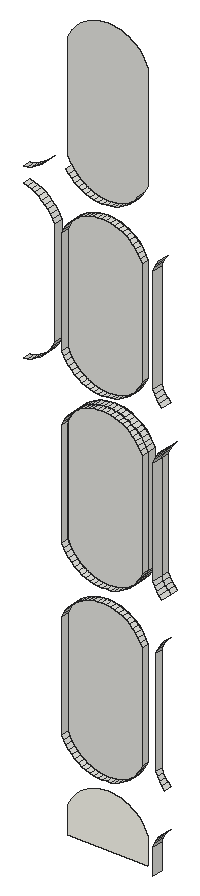
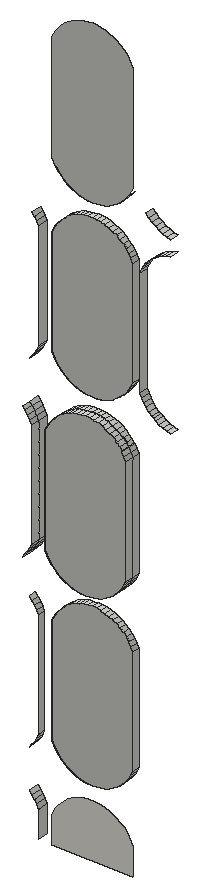
# SketchUp Ruby script. Lengths in inches.
U = 1.inch
M = Sketchup.active_model
def pt(a) = Geom::Point3d.new(a.map { |v| v * U })
def face(e, loops, mat)
  f = e.add_face(loops[0].map { |a| pt(a) })
  loops[1..].each { |l| e.add_face(l.map { |a| pt(a) }).erase! }
  f.material = f.back_material = mat if mat
  f
end
# faces: each face lists its corners as indices into pts; further lists are holes
def faces(e, pts, list, mat = nil) = list.each { |f| face(e, (f[0].is_a?(Array) ? f : [f]).map { |l| l.map { |i| pts[i] } }, mat) }
# xy, xz, yz: faces in a plane at the given z, y or x. An outline is a flat list of corners, or four numbers for a rectangle; further outlines are holes
def ring(l) = l.size == 4 ? [[l[0], l[1]], [l[2], l[1]], [l[2], l[3]], [l[0], l[3]]] : l.each_slice(2).to_a
def flat(e, list, mat, &to3) = list.each { |f| face(e, (f[0].is_a?(Array) ? f : [f]).map { |l| ring(l).map { |u, v| to3.(u, v) } }, mat) }
def xy(e, z, list, mat = nil) = flat(e, list, mat) { |x, y| [x, y, z] }
def xz(e, y, list, mat = nil) = flat(e, list, mat) { |x, z| [x, y, z] }
def yz(e, x, list, mat = nil) = flat(e, list, mat) { |y, z| [x, y, z] }
def lines(e, pts, list) = list.each { |a, b| e.add_line(pt(pts[a]), pt(pts[b])) }
# prism: a flat outline (further loops are holes) pulled along v
def prism(e, loops, v, mat = nil)
  f = face(e, loops, mat); d = Geom::Vector3d.new(v.map { |x| x * U })
  f.pushpull(f.normal.samedirection?(d) ? d.length : -d.length)
end
def box(e, o, s, mat = nil) = prism(e, [[o, [o[0] + s[0], o[1], o[2]], [o[0] + s[0], o[1] + s[1], o[2]], [o[0], o[1] + s[1], o[2]]]], [0, 0, s[2]], mat)
def at(x, y, z, deg = 0) = Geom::Transformation.translation(pt([x, y, z])) * Geom::Transformation.rotation(ORIGIN, Z_AXIS, deg.degrees)
def axes(o, x, y, z) = Geom::Transformation.new([*x, 0, *y, 0, *z, 0, *pt(o).to_a, 1])
def part(name) = M.definitions.add(name)
# library, detail: a bought-in or finely detailed component or shape, given as its bounding box
def library(name, o, s) = part(name).tap { |d| box(d.entities, o, s) }
def detail(e, o, s) = box(e.add_group.entities, o, s)
def put(e, d, t, mat = nil) = e.add_instance(d, t).tap { |i| i.material = mat if mat }
def group(e, t, mat = nil) = e.add_group.tap { |g| g.transformation = t; g.material = mat if mat }.entities
root = M.entities
M.materials.add("Tafisa-Gardenia-or-Gardenia-PM775-4K").color = [246, 245, 235]
xz(root,138.79,[[89.53,11,89.85,11.02,90.17,11.0625,90.48,11.14,90.78,11.25,91.07,11.38,91.35,11.55,91.61,11.73,91.84,11.95,92.0625,12.18,92.25,12.4375,92.42,12.71,92.5625,13,92.5625,21,92.42,21.29,92.25,21.5625,92.0625,21.82,91.84,22.05,91.61,22.27,91.35,22.45,91.07,22.62,90.78,22.75,90.48,22.86,90.17,22.9375,89.85,22.98,89.53,23,89.21,22.98,88.89,22.9375,88.58,22.86,88.28,22.75,87.99,22.62,87.72,22.45,87.46,22.27,87.22,22.05,87,21.82,86.81,21.5625,86.64,21.29,86.5,21,86.5,13,86.64,12.71,86.81,12.4375,87,12.18,87.22,11.95,87.46,11.73,87.72,11.55,87.99,11.38,88.28,11.25,88.58,11.14,88.89,11.0625,89.21,11.02],[89.53,24,89.85,24.02,90.17,24.0625,90.48,24.14,90.78,24.25,91.07,24.38,91.35,24.55,91.61,24.73,91.84,24.95,92.0625,25.18,92.25,25.4375,92.42,25.71,92.5625,26,92.5625,34,92.42,34.29,92.25,34.5625,92.0625,34.82,91.84,35.05,91.61,35.27,91.35,35.45,91.07,35.62,90.78,35.75,90.48,35.86,90.17,35.9375,89.85,35.98,89.53,36,89.21,35.98,88.89,35.9375,88.58,35.86,88.28,35.75,87.99,35.62,87.72,35.45,87.46,35.27,87.22,35.05,87,34.82,86.86,34.63,86.81,34.5625,86.64,34.29,86.5,34,86.5,26,86.64,25.71,86.81,25.4375,87,25.18,87.22,24.95,87.46,24.73,87.72,24.55,87.99,24.38,88.28,24.25,88.58,24.14,88.89,24.0625,89.21,24.02],[89.53,37,89.85,37.02,90.17,37.0625,90.48,37.14,90.78,37.25,91.07,37.38,91.35,37.55,91.61,37.73,91.84,37.95,92.0625,38.18,92.25,38.4375,92.42,38.71,92.5625,39,92.5625,47,92.42,47.29,92.25,47.5625,92.0625,47.82,91.84,48.05,91.61,48.27,91.35,48.45,91.07,48.62,90.78,48.75,90.48,48.86,90.17,48.9375,89.85,48.98,89.53,49,89.21,48.98,88.89,48.9375,88.58,48.86,88.28,48.75,87.99,48.62,87.72,48.45,87.46,48.27,87.22,48.05,87,47.82,86.81,47.5625,86.64,47.29,86.5,47,86.5,39,86.64,38.71,86.81,38.4375,87,38.18,87.22,37.95,87.46,37.73,87.72,37.55,87.99,37.38,88.28,37.25,88.58,37.14,88.89,37.0625,89.21,37.02],[89.53,50,89.85,50.02,90.17,50.0625,90.48,50.14,90.78,50.25,91.07,50.38,91.35,50.55,91.61,50.73,91.84,50.95,92.0625,51.18,92.25,51.4375,92.42,51.71,92.5625,52,92.5625,60,92.42,60.29,92.25,60.5625,92.0625,60.82,91.84,61.05,91.61,61.27,91.35,61.45,91.07,61.62,90.78,61.75,90.48,61.86,90.17,61.9375,89.85,61.98,89.53,62,89.21,61.98,88.89,61.9375,88.58,61.86,88.28,61.75,87.99,61.62,87.72,61.45,87.46,61.27,87.22,61.05,87,60.82,86.81,60.5625,86.64,60.29,86.5,60,86.5,52,86.64,51.71,86.81,51.4375,87,51.18,87.22,50.95,87.46,50.73,87.72,50.55,87.99,50.38,88.28,50.25,88.58,50.14,88.89,50.0625,89.21,50.02]])
xz(root,138.79,[[86.5,6,92.5625,6,92.5625,8,92.42,8.29,92.25,8.5625,92.0625,8.82,91.84,9.05,91.61,9.27,91.35,9.45,91.07,9.62,90.78,9.75,90.48,9.86,90.17,9.9375,89.85,9.98,89.53,10,89.21,9.98,88.89,9.9375,88.58,9.86,88.28,9.75,87.99,9.62,87.72,9.45,87.46,9.27,87.22,9.05,87,8.82,86.81,8.5625,86.64,8.29,86.5,8]],"Tafisa-Gardenia-or-Gardenia-PM775-4K")
xz(root,139.4375,[[89.53,24,89.85,24.02,90.17,24.0625,90.48,24.14,90.78,24.25,91.07,24.38,91.35,24.55,91.61,24.73,91.84,24.95,92.0625,25.18,92.25,25.4375,92.42,25.71,92.5625,26,92.5625,34,92.42,34.29,92.25,34.5625,92.0625,34.82,91.84,35.05,91.61,35.27,91.35,35.45,91.07,35.62,90.78,35.75,90.48,35.86,90.17,35.9375,89.85,35.98,89.53,36,89.21,35.98,88.89,35.9375,88.58,35.86,88.28,35.75,87.99,35.62,87.72,35.45,87.46,35.27,87.22,35.05,87,34.82,86.86,34.63,86.81,34.5625,86.64,34.29,86.5,34,86.5,26,86.64,25.71,86.81,25.4375,87,25.18,87.22,24.95,87.46,24.73,87.72,24.55,87.99,24.38,88.28,24.25,88.58,24.14,88.89,24.0625,89.21,24.02]])
yz(root,85.5,[[138.79,39,139.4375,47]])
yz(root,86.5,[[138.25,13,138.79,21],[138.25,26,138.79,34],[138.79,26,139.4375,34],[138.25,39,138.79,47]])
yz(root,92.5625,[[138.25,13,138.79,21],[138.25,26,138.79,34],[138.79,26,139.4375,34],[138.25,39,138.79,47]])
yz(root,93.5625,[[138,6,138.79,8],[138.25,13,138.79,21],[138,26,138.79,34],[138.79,26,139.4375,34],[138,39,138.79,47]])
p = [[93.5625,138.79,8],[93.7,138.79,8.29],[93.7,138,8.29],[93.5625,138,8],[93.86,138.79,8.56],[93.86,138,8.56],
  [94.04,138.79,8.81],[94.04,138,8.81],[94.25,138.79,9.05],[94.25,138,9.05],[89.21,138.79,11.02],[88.89,138.79,11.0625],
  [88.89,138.25,11.0625],[89.21,138.25,11.02],[89.53,138.79,11],[89.53,138.25,11],[89.85,138.79,11.02],[89.85,138.25,11.02],
  [90.17,138.79,11.0625],[90.17,138.25,11.0625],[88.58,138.79,11.14],[88.28,138.79,11.25],[88.28,138.25,11.25],[88.58,138.25,11.14],
  [90.48,138.79,11.14],[90.48,138.25,11.14],[90.78,138.79,11.25],[90.78,138.25,11.25],[87.99,138.79,11.38],[87.99,138.25,11.38],
  [91.07,138.79,11.38],[91.07,138.25,11.38],[87.72,138.79,11.55],[87.72,138.25,11.55],[91.35,138.79,11.55],[91.35,138.25,11.55],
  [87.46,138.79,11.73],[87.46,138.25,11.73],[91.61,138.79,11.73],[91.61,138.25,11.73],[87.22,138.79,11.95],[87.22,138.25,11.95],
  [91.84,138.79,11.95],[91.84,138.25,11.95],[87,138.79,12.18],[87,138.25,12.18],[92.0625,138.79,12.18],[92.0625,138.25,12.18],
  [94.25,138.79,11.95],[94.04,138.79,12.19],[94.04,138.25,12.19],[94.25,138.25,11.95],[86.81,138.79,12.4375],[86.81,138.25,12.4375],
  [92.25,138.79,12.4375],[92.25,138.25,12.4375],[93.86,138.79,12.44],[93.86,138.25,12.44],[86.64,138.79,12.71],[86.64,138.25,12.71],
  [92.42,138.79,12.71],[92.42,138.25,12.71],[93.7,138.79,12.71],[93.7,138.25,12.71],[86.5,138.79,13],[86.5,138.25,13],
  [92.5625,138.79,13],[92.5625,138.25,13],[93.5625,138.79,13],[93.5625,138.25,13],[86.5,138.79,21],[86.64,138.79,21.29],
  [86.64,138.25,21.29],[86.5,138.25,21],[92.42,138.79,21.29],[92.5625,138.79,21],[92.5625,138.25,21],[92.42,138.25,21.29],
  [93.5625,138.79,21],[93.7,138.79,21.29],[93.7,138.25,21.29],[93.5625,138.25,21],[86.81,138.79,21.5625],[86.81,138.25,21.5625],
  [92.25,138.79,21.5625],[92.25,138.25,21.5625],[93.86,138.79,21.56],[93.86,138.25,21.56],[87,138.79,21.82],[87,138.25,21.82],
  [92.0625,138.79,21.82],[92.0625,138.25,21.82],[94.04,138.79,21.81],[94.04,138.25,21.81],[87.22,138.79,22.05],[87.22,138.25,22.05],
  [91.84,138.79,22.05],[91.84,138.25,22.05],[94.25,138.79,22.05],[94.25,138.25,22.05],[87.46,138.79,22.27],[87.46,138.25,22.27],
  [91.61,138.79,22.27],[91.61,138.25,22.27],[87.72,138.79,22.45],[87.72,138.25,22.45],[91.35,138.79,22.45],[91.35,138.25,22.45],
  [87.99,138.79,22.62],[87.99,138.25,22.62],[91.07,138.79,22.62],[91.07,138.25,22.62],[88.28,138.79,22.75],[88.28,138.25,22.75],
  [90.78,138.79,22.75],[90.78,138.25,22.75],[88.58,138.79,22.86],[88.58,138.25,22.86],[90.48,138.79,22.86],[90.48,138.25,22.86],
  [88.89,138.79,22.9375],[88.89,138.25,22.9375],[89.21,138.79,22.98],[89.21,138.25,22.98],[89.02,138.25,22.96],[89.85,138.79,22.98],
  [90.17,138.79,22.9375],[90.17,138.25,22.9375],[89.85,138.25,22.98],[89.53,138.79,23],[89.53,138.25,23],[89.21,138.79,24.02],
  [88.89,138.79,24.0625],[88.89,138.25,24.0625],[89.02,138.25,24.04],[89.21,138.25,24.02],[89.53,138.79,24],[89.53,138.25,24],
  [89.85,138.79,24.02],[89.85,138.25,24.02],[90.17,138.79,24.0625],[90.17,138.25,24.0625],[88.89,139.4375,24.0625],[89.21,139.4375,24.02],
  [89.53,139.4375,24],[89.85,139.4375,24.02],[90.17,139.4375,24.0625],[88.58,138.79,24.14],[88.28,138.79,24.25],[88.28,138.25,24.25],
  [88.58,138.25,24.14],[90.48,138.79,24.14],[90.48,138.25,24.14],[90.78,138.79,24.25],[90.78,138.25,24.25],[88.28,139.4375,24.25],
  [88.58,139.4375,24.14],[90.48,139.4375,24.14],[90.78,139.4375,24.25],[87.99,138.79,24.38],[87.99,138.25,24.38],[91.07,138.79,24.38],
  [91.07,138.25,24.38],[87.99,139.4375,24.38],[91.07,139.4375,24.38],[87.72,138.79,24.55],[87.72,138.25,24.55],[91.35,138.79,24.55],
  [91.35,138.25,24.55],[87.72,139.4375,24.55],[91.35,139.4375,24.55],[87.46,138.79,24.73],[87.46,138.25,24.73],[91.61,138.79,24.73],
  [91.61,138.25,24.73],[87.46,139.4375,24.73],[91.61,139.4375,24.73],[87.22,138.79,24.95],[87.22,138.25,24.95],[91.84,138.79,24.95],
  [91.84,138.25,24.95],[87.22,139.4375,24.95],[91.84,139.4375,24.95],[94.25,138.79,24.95],[94.04,138.79,25.19],[94.04,138,25.19],
  [94.25,138,24.95],[87,138.79,25.18],[87,138.25,25.18],[92.0625,138.79,25.18],[92.0625,138.25,25.18],[87,139.4375,25.18],
  [92.0625,139.4375,25.18],[94.04,139.4375,25.19],[94.25,139.4375,24.95],[93.86,138.79,25.44],[93.86,138,25.44],[86.81,138.79,25.4375],
  [86.81,138.25,25.4375],[92.25,138.79,25.4375],[92.25,138.25,25.4375],[86.81,139.4375,25.4375],[92.25,139.4375,25.4375],[93.86,139.4375,25.44],
  [93.7,138.79,25.71],[93.7,138,25.71],[86.64,138.79,25.71],[86.64,138.25,25.71],[92.42,138.79,25.71],[92.42,138.25,25.71],
  [86.64,139.4375,25.71],[92.42,139.4375,25.71],[93.7,139.4375,25.71],[93.5625,138.79,26],[93.5625,138,26],[86.5,138.79,26],
  [86.5,138.25,26],[92.5625,138.79,26],[92.5625,138.25,26],[86.5,139.4375,26],[92.5625,139.4375,26],[93.5625,139.4375,26],
  [93.5625,138.79,34],[93.7,138.79,34.29],[93.7,138,34.29],[93.5625,138,34],[86.5,138.79,34],[86.64,138.79,34.29],
  [86.64,138.25,34.29],[86.5,138.25,34],[92.42,138.79,34.29],[92.5625,138.79,34],[92.5625,138.25,34],[92.42,138.25,34.29],
  [86.64,139.4375,34.29],[86.5,139.4375,34],[92.5625,139.4375,34],[92.42,139.4375,34.29],[93.7,139.4375,34.29],[93.5625,139.4375,34],
  [93.86,138.79,34.56],[93.86,138,34.56],[86.81,138.79,34.5625],[86.81,138.25,34.5625],[92.25,138.79,34.5625],[92.25,138.25,34.5625],
  [86.81,139.4375,34.5625],[92.25,139.4375,34.5625],[93.86,139.4375,34.56],[94.04,138.79,34.81],[94.04,138,34.81],[86.86,138.79,34.63],
  [86.86,138.25,34.63],[87,138.79,34.82],[87,138.25,34.82],[92.0625,138.79,34.82],[92.0625,138.25,34.82],[86.86,139.4375,34.63],
  [87,139.4375,34.82],[92.0625,139.4375,34.82],[94.04,139.4375,34.81],[94.25,138.79,35.05],[94.25,138,35.05],[87.22,138.79,35.05],
  [87.22,138.25,35.05],[91.84,138.79,35.05],[91.84,138.25,35.05],[87.22,139.4375,35.05],[91.84,139.4375,35.05],[94.25,139.4375,35.05],
  [87.46,138.79,35.27],[87.46,138.25,35.27],[91.61,138.79,35.27],[91.61,138.25,35.27],[87.46,139.4375,35.27],[91.61,139.4375,35.27],
  [87.72,138.79,35.45],[87.72,138.25,35.45],[91.35,138.79,35.45],[91.35,138.25,35.45],[87.72,139.4375,35.45],[91.35,139.4375,35.45],
  [87.99,138.79,35.62],[87.99,138.25,35.62],[91.07,138.79,35.62],[91.07,138.25,35.62],[87.99,139.4375,35.62],[91.07,139.4375,35.62],
  [88.28,138.79,35.75],[88.28,138.25,35.75],[90.78,138.79,35.75],[90.78,138.25,35.75],[88.28,139.4375,35.75],[90.78,139.4375,35.75],
  [88.58,138.79,35.86],[88.58,138.25,35.86],[90.48,138.79,35.86],[90.48,138.25,35.86],[88.58,139.4375,35.86],[90.48,139.4375,35.86],
  [88.89,138.79,35.9375],[88.89,138.25,35.9375],[89.21,138.79,35.98],[89.21,138.25,35.98],[89.02,138.25,35.96],[89.85,138.79,35.98],
  [90.17,138.79,35.9375],[90.17,138.25,35.9375],[89.85,138.25,35.98],[88.89,139.4375,35.9375],[89.21,139.4375,35.98],[90.17,139.4375,35.9375],
  [89.85,139.4375,35.98],[89.53,138.79,36],[89.53,138.25,36],[89.53,139.4375,36],[89.21,138.79,37.02],[88.89,138.79,37.0625],
  [88.89,138.25,37.0625],[89.02,138.25,37.04],[89.21,138.25,37.02],[89.53,138.79,37],[89.53,138.25,37],[89.85,138.79,37.02],
  [89.85,138.25,37.02],[90.17,138.79,37.0625],[90.17,138.25,37.0625],[88.58,138.79,37.14],[88.28,138.79,37.25],[88.28,138.25,37.25],
  [88.58,138.25,37.14],[90.48,138.79,37.14],[90.48,138.25,37.14],[90.78,138.79,37.25],[90.78,138.25,37.25],[83.13,139.4375,37.0625],
  [83.13,138.79,37.0625],[83.44,138.79,37.14],[83.44,139.4375,37.14],[83.74,138.79,37.25],[83.74,139.4375,37.25],[87.99,138.79,37.38],
  [87.99,138.25,37.38],[91.07,138.79,37.38],[91.07,138.25,37.38],[84.03,138.79,37.38],[84.03,139.4375,37.38],[87.72,138.79,37.55],
  [87.72,138.25,37.55],[91.35,138.79,37.55],[91.35,138.25,37.55],[84.3,138.79,37.55],[84.3,139.4375,37.55],[87.46,138.79,37.73],
  [87.46,138.25,37.73],[91.61,138.79,37.73],[91.61,138.25,37.73],[84.46,138.79,37.66],[84.46,139.4375,37.66],[87.22,138.79,37.95],
  [87.22,138.25,37.95],[91.84,138.79,37.95],[91.84,138.25,37.95],[84.56,138.79,37.74],[84.56,139.4375,37.74],[84.79,138.79,37.95],
  [84.79,139.4375,37.95],[94.25,138.79,37.95],[94.04,138.79,38.19],[94.04,138,38.19],[94.25,138,37.95],[87,138.79,38.18],
  [87,138.25,38.18],[92.0625,138.79,38.18],[92.0625,138.25,38.18],[85.01,138.79,38.18],[85.01,139.4375,38.18],[93.86,138.79,38.44],
  [93.86,138,38.44],[86.81,138.79,38.4375],[86.81,138.25,38.4375],[92.25,138.79,38.4375],[92.25,138.25,38.4375],[85.2,138.79,38.44],
  [85.2,139.4375,38.44],[93.7,138.79,38.71],[93.7,138,38.71],[86.64,138.79,38.71],[86.64,138.25,38.71],[92.42,138.79,38.71],
  [92.42,138.25,38.71],[85.36,138.79,38.71],[85.36,139.4375,38.71],[93.5625,138.79,39],[93.5625,138,39],[86.5,138.79,39],
  [86.5,138.25,39],[92.5625,138.79,39],[92.5625,138.25,39],[85.5,138.79,39],[85.5,139.4375,39],[93.5625,138.79,47],
  [93.7,138.79,47.29],[93.7,138,47.29],[93.5625,138,47],[86.5,138.79,47],[86.64,138.79,47.29],[86.64,138.25,47.29],
  [86.5,138.25,47],[92.42,138.79,47.29],[92.5625,138.79,47],[92.5625,138.25,47],[92.42,138.25,47.29],[85.5,139.4375,47],
  [85.5,138.79,47],[85.36,138.79,47.29],[85.36,139.4375,47.29],[93.86,138.79,47.56],[93.86,138,47.56],[86.81,138.79,47.5625],
  [86.81,138.25,47.5625],[92.25,138.79,47.5625],[92.25,138.25,47.5625],[85.2,138.79,47.56],[85.2,139.4375,47.56],[94.04,138.79,47.81],
  [94.04,138,47.81],[87,138.79,47.82],[87,138.25,47.82],[92.0625,138.79,47.82],[92.0625,138.25,47.82],[85.01,138.79,47.82],
  [85.01,139.4375,47.82],[87.22,138.79,48.05],[87.22,138.25,48.05],[91.84,138.79,48.05],[91.84,138.25,48.05],[84.79,138.79,48.05],
  [84.79,139.4375,48.05],[87.46,138.79,48.27],[87.46,138.25,48.27],[91.61,138.79,48.27],[91.61,138.25,48.27],[84.56,138.79,48.26],
  [84.56,139.4375,48.26],[87.72,138.79,48.45],[87.72,138.25,48.45],[91.35,138.79,48.45],[91.35,138.25,48.45],[84.3,138.79,48.45],
  [84.3,139.4375,48.45],[87.99,138.79,48.62],[87.99,138.25,48.62],[91.07,138.79,48.62],[91.07,138.25,48.62],[84.03,138.79,48.62],
  [84.03,139.4375,48.62],[88.28,138.79,48.75],[88.28,138.25,48.75],[90.78,138.79,48.75],[90.78,138.25,48.75],[83.74,138.79,48.75],
  [83.74,139.4375,48.75],[88.58,138.79,48.86],[88.58,138.25,48.86],[90.48,138.79,48.86],[90.48,138.25,48.86],[83.44,138.79,48.86],
  [83.44,139.4375,48.86],[88.89,138.79,48.9375],[88.89,138.25,48.9375],[89.21,138.79,48.98],[89.21,138.25,48.98],[89.02,138.25,48.96],
  [89.85,138.79,48.98],[90.17,138.79,48.9375],[90.17,138.25,48.9375],[89.85,138.25,48.98],[83.13,138.79,48.9375],[83.13,139.4375,48.9375],
  [89.53,138.79,49],[89.53,138.25,49],[89.21,138.79,50.02],[88.89,138.79,50.0625],[88.89,138.25,50.0625],[89.02,138.25,50.04],
  [89.21,138.25,50.02],[89.53,138.79,50],[89.53,138.25,50],[89.85,138.79,50.02],[89.85,138.25,50.02],[90.17,138.79,50.0625],
  [90.17,138.25,50.0625],[88.58,138.79,50.14],[88.28,138.79,50.25],[88.28,138.25,50.25],[88.58,138.25,50.14],[90.48,138.79,50.14],
  [90.48,138.25,50.14],[90.78,138.79,50.25],[90.78,138.25,50.25],[83.13,139.4375,50.0625],[83.13,138.79,50.0625],[83.44,138.79,50.14],
  [83.44,139.4375,50.14],[83.74,138.79,50.25],[83.74,139.4375,50.25],[87.99,138.79,50.38],[87.99,138.25,50.38],[91.07,138.79,50.38],
  [91.07,138.25,50.38],[84.03,138.79,50.38],[84.03,139.4375,50.38],[87.72,138.79,50.55],[87.72,138.25,50.55],[91.35,138.79,50.55],
  [91.35,138.25,50.55],[84.3,138.79,50.55],[84.3,139.4375,50.55],[87.46,138.79,50.73],[87.46,138.25,50.73],[91.61,138.79,50.73],
  [91.61,138.25,50.73],[84.56,138.79,50.74],[84.56,139.4375,50.74],[87.22,138.79,50.95],[87.22,138.25,50.95],[91.84,138.79,50.95],
  [91.84,138.25,50.95],[84.79,138.79,50.95],[84.79,139.4375,50.95],[87,138.79,51.18],[87,138.25,51.18],[92.0625,138.79,51.18],
  [92.0625,138.25,51.18],[85.01,138.79,51.18],[85.01,139.4375,51.18],[86.81,138.79,51.4375],[86.81,138.25,51.4375],[92.25,138.79,51.4375],
  [92.25,138.25,51.4375]]
faces(root,p,[[0,1,2,3],[1,4,5,2],[4,6,7,5],[6,8,9,7],[10,11,12,13],[14,10,13,15],[16,14,15,17],[18,16,17,19],
  [20,21,22,23],[11,20,23,12],[24,18,19,25],[26,24,25,27],[21,28,29,22],[30,26,27,31],[28,32,33,29],[34,30,31,35],
  [32,36,37,33],[38,34,35,39],[36,40,41,37],[42,38,39,43],[40,44,45,41],[46,42,43,47],[48,49,50,51],[44,52,53,45],
  [54,46,47,55],[49,56,57,50],[52,58,59,53],[60,54,55,61],[56,62,63,57],[58,64,65,59],[66,60,61,67],[62,68,69,63],
  [70,71,72,73],[74,75,76,77],[78,79,80,81],[71,82,83,72],[84,74,77,85],[79,86,87,80],[82,88,89,83],[90,84,85,91],
  [86,92,93,87],[88,94,95,89],[96,90,91,97],[92,98,99,93],[94,100,101,95],[102,96,97,103],[100,104,105,101],[106,102,103,107],
  [104,108,109,105],[110,106,107,111],[108,112,113,109],[114,110,111,115],[112,116,117,113],[118,114,115,119],[116,120,121,117],[120,122,123,124,121],
  [125,126,127,128],[126,118,119,127],[122,129,130,123],[129,125,128,130],[131,132,133,134,135],[136,131,135,137],[138,136,137,139],[140,138,139,141],
  [142,132,131,143],[143,131,136,144],[144,136,138,145],[145,138,140,146],[147,148,149,150],[132,147,150,133],[151,140,141,152],[153,151,152,154],
  [155,148,147,156],[156,147,132,142],[146,140,151,157],[157,151,153,158],[148,159,160,149],[161,153,154,162],[163,159,148,155],[158,153,161,164],
  [159,165,166,160],[167,161,162,168],[169,165,159,163],[164,161,167,170],[165,171,172,166],[173,167,168,174],[175,171,165,169],[170,167,173,176],
  [171,177,178,172],[179,173,174,180],[181,177,171,175],[176,173,179,182],[183,184,185,186],[177,187,188,178],[189,179,180,190],[191,187,177,181],
  [182,179,189,192],[193,184,183,194],[184,195,196,185],[187,197,198,188],[199,189,190,200],[201,197,187,191],[192,189,199,202],[203,195,184,193],
  [195,204,205,196],[197,206,207,198],[208,199,200,209],[210,206,197,201],[202,199,208,211],[212,204,195,203],[204,213,214,205],[206,215,216,207],
  [217,208,209,218],[219,215,206,210],[211,208,217,220],[221,213,204,212],[222,223,224,225],[226,227,228,229],[230,231,232,233],[234,227,226,235],
  [236,231,230,237],[238,223,222,239],[223,240,241,224],[227,242,243,228],[244,230,233,245],[246,242,227,234],[237,230,244,247],[248,240,223,238],
  [240,249,250,241],[242,251,252,243],[253,254,252,251],[255,244,245,256],[257,251,242,246],[258,253,251,257],[247,244,255,259],[260,249,240,248],
  [249,261,262,250],[253,263,264,254],[265,255,256,266],[267,263,253,258],[259,255,265,268],[269,261,249,260],[263,270,271,264],[272,265,266,273],
  [274,270,263,267],[268,265,272,275],[270,276,277,271],[278,272,273,279],[280,276,270,274],[275,272,278,281],[276,282,283,277],[284,278,279,285],
  [286,282,276,280],[281,278,284,287],[282,288,289,283],[290,284,285,291],[292,288,282,286],[287,284,290,293],[288,294,295,289],[296,290,291,297],
  [298,294,288,292],[293,290,296,299],[294,300,301,295],[300,302,303,304,301],[305,306,307,308],[306,296,297,307],[309,300,294,298],[310,302,300,309],
  [311,306,305,312],[299,296,306,311],[302,313,314,303],[313,305,308,314],[315,313,302,310],[312,305,313,315],[316,317,318,319,320],[321,316,320,322],
  [323,321,322,324],[325,323,324,326],[327,328,329,330],[317,327,330,318],[331,325,326,332],[333,331,332,334],[335,336,337,338],[338,337,339,340],
  [328,341,342,329],[343,333,334,344],[340,339,345,346],[341,347,348,342],[349,343,344,350],[346,345,351,352],[347,353,354,348],[355,349,350,356],
  [352,351,357,358],[353,359,360,354],[361,355,356,362],[358,357,363,364],[364,363,365,366],[367,368,369,370],[359,371,372,360],[373,361,362,374],
  [366,365,375,376],[368,377,378,369],[371,379,380,372],[381,373,374,382],[376,375,383,384],[377,385,386,378],[379,387,388,380],[389,381,382,390],
  [384,383,391,392],[385,393,394,386],[387,395,396,388],[397,389,390,398],[392,391,399,400],[401,402,403,404],[405,406,407,408],[409,410,411,412],
  [413,414,415,416],[402,417,418,403],[406,419,420,407],[421,409,412,422],[416,415,423,424],[417,425,426,418],[419,427,428,420],[429,421,422,430],
  [424,423,431,432],[427,433,434,428],[435,429,430,436],[432,431,437,438],[433,439,440,434],[441,435,436,442],[438,437,443,444],[439,445,446,440],
  [447,441,442,448],[444,443,449,450],[445,451,452,446],[453,447,448,454],[450,449,455,456],[451,457,458,452],[459,453,454,460],[456,455,461,462],
  [457,463,464,458],[465,459,460,466],[462,461,467,468],[463,469,470,464],[469,471,472,473,470],[474,475,476,477],[475,465,466,476],[468,467,478,479],
  [471,480,481,472],[480,474,477,481],[482,483,484,485,486],[487,482,486,488],[489,487,488,490],[491,489,490,492],[493,494,495,496],[483,493,496,484],
  [497,491,492,498],[499,497,498,500],[501,502,503,504],[504,503,505,506],[494,507,508,495],[509,499,500,510],[506,505,511,512],[507,513,514,508],
  [515,509,510,516],[512,511,517,518],[513,519,520,514],[521,515,516,522],[518,517,523,524],[519,525,526,520],[527,521,522,528],[524,523,529,530],
  [525,531,532,526],[533,527,528,534],[530,529,535,536],[531,537,538,532],[539,533,534,540]])
